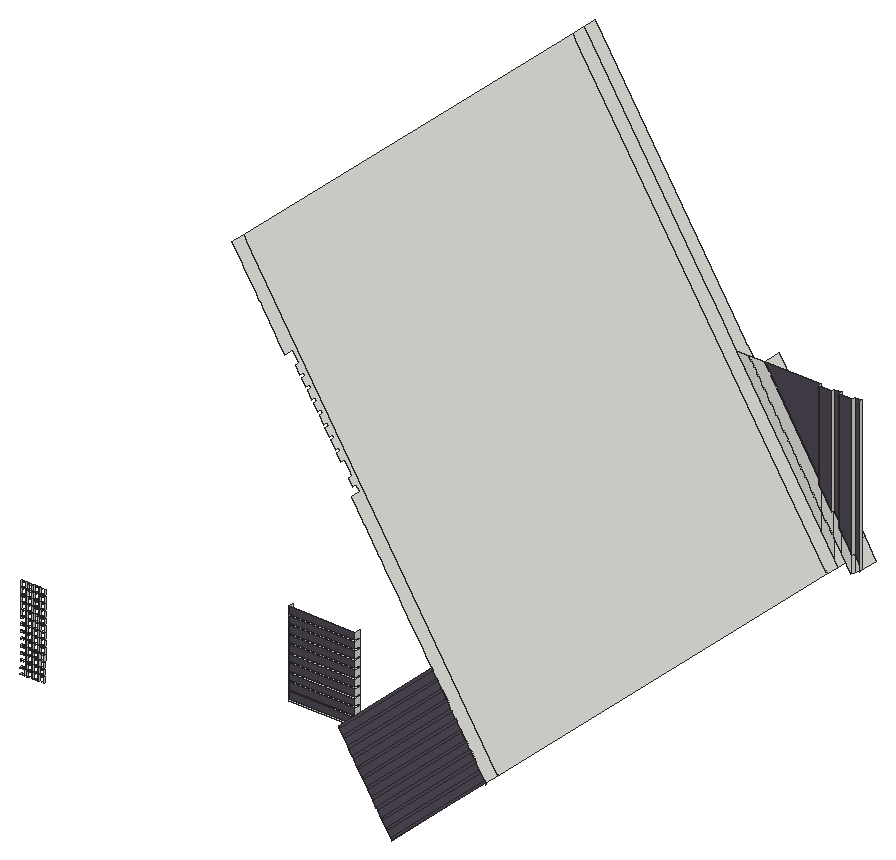
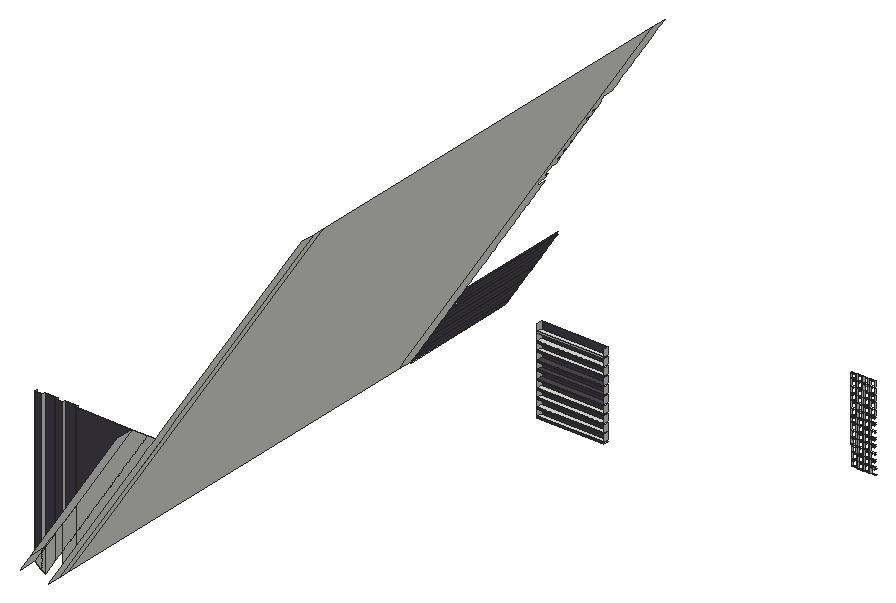
# SketchUp Ruby script. Lengths in inches.
U = 1.inch
M = Sketchup.active_model
def pt(a) = Geom::Point3d.new(a.map { |v| v * U })
def face(e, loops, mat)
  f = e.add_face(loops[0].map { |a| pt(a) })
  loops[1..].each { |l| e.add_face(l.map { |a| pt(a) }).erase! }
  f.material = f.back_material = mat if mat
  f
end
# faces: each face lists its corners as indices into pts; further lists are holes
def faces(e, pts, list, mat = nil) = list.each { |f| face(e, (f[0].is_a?(Array) ? f : [f]).map { |l| l.map { |i| pts[i] } }, mat) }
# xy, xz, yz: faces in a plane at the given z, y or x. An outline is a flat list of corners, or four numbers for a rectangle; further outlines are holes
def ring(l) = l.size == 4 ? [[l[0], l[1]], [l[2], l[1]], [l[2], l[3]], [l[0], l[3]]] : l.each_slice(2).to_a
def flat(e, list, mat, &to3) = list.each { |f| face(e, (f[0].is_a?(Array) ? f : [f]).map { |l| ring(l).map { |u, v| to3.(u, v) } }, mat) }
def xy(e, z, list, mat = nil) = flat(e, list, mat) { |x, y| [x, y, z] }
def xz(e, y, list, mat = nil) = flat(e, list, mat) { |x, z| [x, y, z] }
def yz(e, x, list, mat = nil) = flat(e, list, mat) { |y, z| [x, y, z] }
def lines(e, pts, list) = list.each { |a, b| e.add_line(pt(pts[a]), pt(pts[b])) }
# prism: a flat outline (further loops are holes) pulled along v
def prism(e, loops, v, mat = nil)
  f = face(e, loops, mat); d = Geom::Vector3d.new(v.map { |x| x * U })
  f.pushpull(f.normal.samedirection?(d) ? d.length : -d.length)
end
def box(e, o, s, mat = nil) = prism(e, [[o, [o[0] + s[0], o[1], o[2]], [o[0] + s[0], o[1] + s[1], o[2]], [o[0], o[1] + s[1], o[2]]]], [0, 0, s[2]], mat)
def at(x, y, z, deg = 0) = Geom::Transformation.translation(pt([x, y, z])) * Geom::Transformation.rotation(ORIGIN, Z_AXIS, deg.degrees)
def axes(o, x, y, z) = Geom::Transformation.new([*x, 0, *y, 0, *z, 0, *pt(o).to_a, 1])
def part(name) = M.definitions.add(name)
# library, detail: a bought-in or finely detailed component or shape, given as its bounding box
def library(name, o, s) = part(name).tap { |d| box(d.entities, o, s) }
def detail(e, o, s) = box(e.add_group.entities, o, s)
def put(e, d, t, mat = nil) = e.add_instance(d, t).tap { |i| i.material = mat if mat }
def group(e, t, mat = nil) = e.add_group.tap { |g| g.transformation = t; g.material = mat if mat }.entities
root = M.entities
M.materials.add("[Color M06]").color = [79, 71, 84]
xy(root,265.77,[[1006.85,2332.13,1009.17,2332.76],[1009.76,2332.13,1012.08,2332.76],[1012.68,2332.13,1014.99,2332.76],[1015.59,2332.13,1017.9,2332.76]])
xy(root,267.02,[[1096.79,2375.74,1127.76,2378.12]])
xy(root,267.83,[[1096.79,2375.74,1127.76,2378.12]])
xy(root,268.09,[[1006.85,2332.13,1009.17,2332.76],[1009.76,2332.13,1012.08,2332.76],[1012.68,2332.13,1014.99,2332.76],[1015.59,2332.13,1017.9,2332.76]])
xy(root,268.82,[[1006.88,2332.13,1009.19,2332.76],[1009.79,2332.13,1012.11,2332.76],[1012.71,2332.13,1015.02,2332.76],[1015.62,2332.13,1017.93,2332.76]])
xy(root,270.95,[[1096.79,2375.74,1127.76,2378.12]])
xy(root,271.13,[[1006.88,2332.13,1009.19,2332.76],[1009.79,2332.13,1012.11,2332.76],[1012.71,2332.13,1015.02,2332.76],[1015.62,2332.13,1017.93,2332.76]])
xy(root,271.76,[[1096.79,2375.74,1127.76,2378.12]])
xy(root,271.86,[[1006.91,2332.13,1009.22,2332.76],[1009.82,2332.13,1012.14,2332.76],[1012.73,2332.13,1015.05,2332.76],[1015.65,2332.13,1017.96,2332.76]])
xy(root,274.17,[[1006.91,2332.13,1009.22,2332.76],[1009.82,2332.13,1012.14,2332.76],[1012.73,2332.13,1015.05,2332.76],[1015.65,2332.13,1017.96,2332.76]])
xy(root,274.89,[[1096.79,2375.74,1127.76,2378.12]])
xy(root,274.91,[[1006.94,2332.13,1009.25,2332.76],[1009.85,2332.13,1012.16,2332.76],[1012.76,2332.13,1015.08,2332.76],[1015.68,2332.13,1017.99,2332.76]])
xy(root,275.7,[[1096.79,2375.74,1127.76,2378.12]])
xy(root,277.22,[[1006.94,2332.13,1009.25,2332.76],[1009.85,2332.13,1012.16,2332.76],[1012.76,2332.13,1015.08,2332.76],[1015.68,2332.13,1017.99,2332.76]])
xy(root,277.95,[[1006.97,2332.13,1009.28,2332.76],[1009.88,2332.13,1012.19,2332.76],[1012.79,2332.13,1015.11,2332.76],[1015.7,2332.13,1018.02,2332.76]])
xy(root,278.83,[[1096.79,2375.74,1127.76,2378.12]])
xy(root,279.64,[[1096.79,2375.74,1127.76,2378.12]])
xy(root,280.26,[[1006.97,2332.13,1009.28,2332.76],[1009.88,2332.13,1012.19,2332.76],[1012.79,2332.13,1015.11,2332.76],[1015.7,2332.13,1018.02,2332.76]])
xy(root,281,[[1007,2332.13,1009.31,2332.76],[1009.91,2332.13,1012.22,2332.76],[1012.82,2332.13,1015.13,2332.76],[1015.73,2332.13,1018.05,2332.76]])
xy(root,282.77,[[1096.79,2375.74,1127.76,2378.12]])
xy(root,283.31,[[1007,2332.13,1009.31,2332.76],[1009.91,2332.13,1012.22,2332.76],[1012.82,2332.13,1015.13,2332.76],[1015.73,2332.13,1018.05,2332.76]])
xy(root,283.58,[[1096.79,2375.74,1127.76,2378.12]],"[Color M06]")
xy(root,284.04,[[1007.03,2332.13,1009.34,2332.76],[1009.9375,2332.13,1012.25,2332.76],[1012.85,2332.13,1015.16,2332.76],[1015.76,2332.13,1018.08,2332.76]])
xy(root,286.35,[[1007.03,2332.13,1009.34,2332.76],[1009.9375,2332.13,1012.25,2332.76],[1012.85,2332.13,1015.16,2332.76],[1015.76,2332.13,1018.08,2332.76]])
xy(root,286.7,[[1096.79,2375.74,1127.76,2378.12]])
xy(root,287.09,[[1007.06,2332.13,1009.37,2332.76],[1009.97,2332.13,1012.28,2332.76],[1012.88,2332.13,1015.19,2332.76],[1015.79,2332.13,1018.1,2332.76]])
xy(root,287.51,[[1096.79,2375.74,1127.76,2378.12]],"[Color M06]")
xy(root,289.4,[[1007.06,2332.13,1009.37,2332.76],[1009.97,2332.13,1012.28,2332.76],[1012.88,2332.13,1015.19,2332.76],[1015.79,2332.13,1018.1,2332.76]])
xy(root,290.13,[[1007.08,2332.13,1009.4,2332.76],[1010,2332.13,1012.31,2332.76],[1012.91,2332.13,1015.22,2332.76],[1015.82,2332.13,1018.13,2332.76]])
xy(root,290.64,[[1096.79,2375.74,1127.76,2378.12]])
xy(root,291.45,[[1096.79,2375.74,1127.76,2378.12]],"[Color M06]")
xy(root,292.44,[[1007.08,2332.13,1009.4,2332.76],[1010,2332.13,1012.31,2332.76],[1012.91,2332.13,1015.22,2332.76],[1015.82,2332.13,1018.13,2332.76]])
xy(root,293.18,[[1007.11,2332.13,1009.43,2332.76],[1010.03,2332.13,1012.34,2332.76],[1012.9375,2332.13,1015.25,2332.76],[1015.85,2332.13,1018.16,2332.76]])
xy(root,294.58,[[1096.79,2375.74,1127.76,2378.12]])
xy(root,295.39,[[1096.79,2375.74,1127.76,2378.12]])
xy(root,295.49,[[1007.11,2332.13,1009.43,2332.76],[1010.03,2332.13,1012.34,2332.76],[1012.9375,2332.13,1015.25,2332.76],[1015.85,2332.13,1018.16,2332.76]])
xy(root,296.22,[[1007.14,2332.13,1009.46,2332.76],[1010.05,2332.13,1012.37,2332.76],[1012.97,2332.13,1015.28,2332.76],[1015.88,2332.13,1018.19,2332.76]])
xy(root,298.52,[[1096.79,2375.74,1127.76,2378.12]])
xy(root,298.53,[[1007.14,2332.13,1009.46,2332.76],[1010.05,2332.13,1012.37,2332.76],[1012.97,2332.13,1015.28,2332.76],[1015.88,2332.13,1018.19,2332.76]])
xy(root,299.27,[[1007.17,2332.13,1009.48,2332.76],[1010.08,2332.13,1012.4,2332.76],[1013,2332.13,1015.31,2332.76],[1015.91,2332.13,1018.22,2332.76]])
xy(root,299.33,[[1096.79,2375.74,1127.76,2378.12]])
xy(root,301.58,[[1007.17,2332.13,1009.48,2332.76],[1010.08,2332.13,1012.4,2332.76],[1013,2332.13,1015.31,2332.76],[1015.91,2332.13,1018.22,2332.76]])
xy(root,302.31,[[1007.2,2332.13,1009.51,2332.76],[1010.11,2332.13,1012.43,2332.76],[1013.02,2332.13,1015.34,2332.76],[1015.9375,2332.13,1018.25,2332.76]])
xy(root,302.45,[[1096.79,2375.74,1127.76,2378.12]])
xy(root,303.26,[[1096.79,2375.74,1127.76,2378.12]])
xy(root,304.62,[[1007.2,2332.13,1009.51,2332.76],[1010.11,2332.13,1012.43,2332.76],[1013.02,2332.13,1015.34,2332.76],[1015.9375,2332.13,1018.25,2332.76]])
xz(root,2373.56,[[1190.19,265.95,1189.93,266.36,1190.19,266.53],[1189.4,267.19,1189.66,267.36,1187.96,270,1187.7,269.84],[1187.17,270.67,1187.43,270.83,1185.74,273.48,1185.48,273.31],[1184.94,274.14,1185.21,274.31,1183.51,276.95,1183.25,276.78],[1182.72,277.61,1182.98,277.78,1181.29,280.42,1181.02,280.25],
  [1180.49,281.08,1180.75,281.25,1179.06,283.89,1178.8,283.73],[1178.26,284.56,1178.53,284.72,1176.83,287.37,1176.57,287.2],[1176.04,288.03,1176.3,288.2,1174.61,290.84,1174.34,290.67],[1173.8125,291.5,1172.12,294.14,1172.38,294.3125,1174.07,291.67],[1171.59,294.97,1171.85,295.14,1170.15,297.79,1169.89,297.62],
  [1169.36,298.45,1169.62,298.61,1167.93,301.26,1167.66,301.09],[1167.03,301.85,1167.4,302.09,1165.7,304.73,1165.33,304.49]])
xz(root,2375.74,[[1096.79,267.83,1127.76,270.95],[1096.79,271.76,1127.76,274.89],[1096.79,275.7,1127.76,278.83],[1096.79,279.64,1127.76,282.77],[1096.79,283.58,1127.76,286.7],
  [1096.79,287.51,1127.76,290.64],[1096.79,291.45,1127.76,294.58],[1096.79,295.39,1127.76,298.52],[1096.79,299.33,1127.76,302.45],[1096.79,303.26,1127.76,306.39]],"[Color M06]")
xz(root,2378.12,[[1096.79,302.45,1127.76,303.26]])
xz(root,2378.12,[[1096.79,267.02,1127.76,267.83],[1096.79,270.95,1127.76,271.76],[1096.79,274.89,1127.76,275.7],[1096.79,278.83,1127.76,279.64],[1096.79,282.77,1127.76,283.58],
  [1096.79,286.7,1127.76,287.51],[1096.79,290.64,1127.76,291.45],[1096.79,294.58,1127.76,295.39],[1096.79,298.52,1127.76,299.33]],"[Color M06]")
xz(root,2576.81,[[1198,274.85,1198,340.125,1191.92,340.125,1191.92,284.33,1196.26,277.56],[1188.5,289.67,1188.5,340.125,1182.42,340.125,1182.42,299.15]],"[Color M06]")
xz(root,2578.12,[[1196.26,265.98,1196.26,277.56,1191.92,284.33,1191.92,272.75],[1196.26,265.98,1198,267.09,1198,274.85,1196.26,277.56],[1198,267.09,1198,274.85,1201.42,269.51,1201.42,269.29],[1188.5,269.17,1188.5,278.09,1182.42,287.57,1182.42,278.65],[1201.42,269.29,1201.52,269.35,1201.42,269.51],
  [1191.92,272.75,1191.92,284.33,1188.5,289.67,1188.5,278.09],[1188.5,278.09,1188.5,289.67,1182.42,299.15,1182.42,287.57],[1182.42,278.65,1182.42,287.57,1148.73,340.125,1143.01,340.125],[1182.42,287.57,1182.42,299.15,1156.15,340.125,1148.73,340.125]])
xz(root,2578.12,[[1201.42,269.51,1201.42,340.125,1198,340.125,1198,274.85],[1191.92,284.33,1191.92,340.125,1188.5,340.125,1188.5,289.67],[1182.42,299.15,1182.42,340.125,1156.15,340.125]],"[Color M06]")
yz(root,1007.08,[[2332.13,290.13,2332.76,292.44]])
yz(root,1007.11,[[2332.13,293.18,2332.76,295.49]])
yz(root,1007.14,[[2332.13,296.22,2332.76,298.53]])
yz(root,1007.17,[[2332.13,299.27,2332.76,301.58]])
yz(root,1007.2,[[2332.13,302.31,2332.76,304.62]])
yz(root,1009.17,[[2332.13,265.77,2332.76,268.09]])
yz(root,1009.19,[[2332.13,268.82,2332.76,271.13]])
yz(root,1009.22,[[2332.13,271.86,2332.76,274.17]])
yz(root,1009.25,[[2332.13,274.91,2332.76,277.22]])
yz(root,1009.28,[[2332.13,277.95,2332.76,280.26]])
yz(root,1009.31,[[2332.13,281,2332.76,283.31]])
yz(root,1009.34,[[2332.13,284.04,2332.76,286.35]])
yz(root,1009.37,[[2332.13,287.09,2332.76,289.4]])
yz(root,1009.4,[[2332.13,290.13,2332.76,292.44]])
yz(root,1009.43,[[2332.13,293.18,2332.76,295.49]])
yz(root,1009.46,[[2332.13,296.22,2332.76,298.53]])
yz(root,1009.48,[[2332.13,299.27,2332.76,301.58]])
yz(root,1009.51,[[2332.13,302.31,2332.76,304.62]])
yz(root,1009.76,[[2332.13,265.77,2332.76,268.09]])
yz(root,1009.79,[[2332.13,268.82,2332.76,271.13]])
yz(root,1009.82,[[2332.13,271.86,2332.76,274.17]])
yz(root,1009.85,[[2332.13,274.91,2332.76,277.22]])
yz(root,1009.88,[[2332.13,277.95,2332.76,280.26]])
yz(root,1009.91,[[2332.13,281,2332.76,283.31]])
yz(root,1009.9375,[[2332.13,284.04,2332.76,286.35]])
yz(root,1009.97,[[2332.13,287.09,2332.76,289.4]])
yz(root,1010,[[2332.13,290.13,2332.76,292.44]])
yz(root,1010.03,[[2332.13,293.18,2332.76,295.49]])
yz(root,1010.05,[[2332.13,296.22,2332.76,298.53]])
yz(root,1010.08,[[2332.13,299.27,2332.76,301.58]])
yz(root,1010.11,[[2332.13,302.31,2332.76,304.62]])
yz(root,1012.08,[[2332.13,265.77,2332.76,268.09]])
yz(root,1012.11,[[2332.13,268.82,2332.76,271.13]])
yz(root,1012.14,[[2332.13,271.86,2332.76,274.17]])
yz(root,1012.16,[[2332.13,274.91,2332.76,277.22]])
yz(root,1012.19,[[2332.13,277.95,2332.76,280.26]])
yz(root,1012.22,[[2332.13,281,2332.76,283.31]])
yz(root,1012.25,[[2332.13,284.04,2332.76,286.35]])
yz(root,1012.28,[[2332.13,287.09,2332.76,289.4]])
yz(root,1012.31,[[2332.13,290.13,2332.76,292.44]])
yz(root,1012.34,[[2332.13,293.18,2332.76,295.49]])
yz(root,1012.37,[[2332.13,296.22,2332.76,298.53]])
yz(root,1012.4,[[2332.13,299.27,2332.76,301.58]])
yz(root,1012.43,[[2332.13,302.31,2332.76,304.62]])
yz(root,1012.68,[[2332.13,265.77,2332.76,268.09]])
yz(root,1012.71,[[2332.13,268.82,2332.76,271.13]])
yz(root,1012.73,[[2332.13,271.86,2332.76,274.17]])
yz(root,1012.76,[[2332.13,274.91,2332.76,277.22]])
yz(root,1012.79,[[2332.13,277.95,2332.76,280.26]])
yz(root,1012.82,[[2332.13,281,2332.76,283.31]])
yz(root,1012.85,[[2332.13,284.04,2332.76,286.35]])
yz(root,1012.88,[[2332.13,287.09,2332.76,289.4]])
yz(root,1012.91,[[2332.13,290.13,2332.76,292.44]])
yz(root,1012.9375,[[2332.13,293.18,2332.76,295.49]])
yz(root,1012.97,[[2332.13,296.22,2332.76,298.53]])
yz(root,1013,[[2332.13,299.27,2332.76,301.58]])
yz(root,1013.02,[[2332.13,302.31,2332.76,304.62]])
yz(root,1014.99,[[2332.13,265.77,2332.76,268.09]])
yz(root,1015.02,[[2332.13,268.82,2332.76,271.13]])
yz(root,1015.05,[[2332.13,271.86,2332.76,274.17]])
yz(root,1015.08,[[2332.13,274.91,2332.76,277.22]])
yz(root,1015.11,[[2332.13,277.95,2332.76,280.26]])
yz(root,1015.13,[[2332.13,281,2332.76,283.31]])
yz(root,1015.16,[[2332.13,284.04,2332.76,286.35]])
yz(root,1015.19,[[2332.13,287.09,2332.76,289.4]])
yz(root,1015.22,[[2332.13,290.13,2332.76,292.44]])
yz(root,1015.25,[[2332.13,293.18,2332.76,295.49]])
yz(root,1015.28,[[2332.13,296.22,2332.76,298.53]])
yz(root,1015.31,[[2332.13,299.27,2332.76,301.58]])
yz(root,1015.34,[[2332.13,302.31,2332.76,304.62]])
yz(root,1015.59,[[2332.13,265.77,2332.76,268.09]])
yz(root,1015.62,[[2332.13,268.82,2332.76,271.13]])
yz(root,1015.65,[[2332.13,271.86,2332.76,274.17]])
yz(root,1015.68,[[2332.13,274.91,2332.76,277.22]])
yz(root,1015.7,[[2332.13,277.95,2332.76,280.26]])
yz(root,1015.73,[[2332.13,281,2332.76,283.31]])
yz(root,1015.76,[[2332.13,284.04,2332.76,286.35]])
yz(root,1015.79,[[2332.13,287.09,2332.76,289.4]])
yz(root,1015.82,[[2332.13,290.13,2332.76,292.44]])
yz(root,1015.85,[[2332.13,293.18,2332.76,295.49]])
yz(root,1015.88,[[2332.13,296.22,2332.76,298.53]])
yz(root,1015.91,[[2332.13,299.27,2332.76,301.58]])
yz(root,1015.9375,[[2332.13,302.31,2332.76,304.62]])
yz(root,1017.9,[[2332.13,265.77,2332.76,268.09]])
yz(root,1017.93,[[2332.13,268.82,2332.76,271.13]])
yz(root,1017.96,[[2332.13,271.86,2332.76,274.17]])
yz(root,1017.99,[[2332.13,274.91,2332.76,277.22]])
yz(root,1018.02,[[2332.13,277.95,2332.76,280.26]])
yz(root,1018.05,[[2332.13,281,2332.76,283.31]])
yz(root,1018.08,[[2332.13,284.04,2332.76,286.35]])
yz(root,1018.1,[[2332.13,287.09,2332.76,289.4]])
yz(root,1018.13,[[2332.13,290.13,2332.76,292.44]])
yz(root,1018.16,[[2332.13,293.18,2332.76,295.49]])
yz(root,1018.19,[[2332.13,296.22,2332.76,298.53]])
yz(root,1018.22,[[2332.13,299.27,2332.76,301.58]])
yz(root,1018.25,[[2332.13,302.31,2332.76,304.62]])
yz(root,1096.79,[[2375.74,267.83,2378.12,270.95],[2375.74,271.76,2378.12,274.89],[2375.74,275.7,2378.12,278.83],[2375.74,279.64,2378.12,282.77],[2375.74,283.58,2378.12,286.7],
  [2375.74,287.51,2378.12,290.64],[2375.74,291.45,2378.12,294.58],[2375.74,295.39,2378.12,298.52],[2375.74,299.33,2378.12,302.45],[2375.74,303.26,2378.12,306.39]])
yz(root,1127.76,[[2375.74,267.83,2378.12,270.95],[2375.74,271.76,2378.12,274.89],[2375.74,275.7,2378.12,278.83],[2375.74,279.64,2378.12,282.77],[2375.74,283.58,2378.12,286.7],
  [2375.74,287.51,2378.12,290.64],[2375.74,291.45,2378.12,294.58],[2375.74,295.39,2378.12,298.52],[2375.74,299.33,2378.12,302.45],[2375.74,303.26,2378.12,306.39]])
yz(root,1182.42,[[2576.81,299.15,2578.12,340.125]])
yz(root,1188.5,[[2576.81,289.67,2578.12,340.125]])
yz(root,1191.92,[[2576.81,284.33,2578.12,340.125]])
yz(root,1198,[[2576.81,274.85,2578.12,340.125]])
yz(root,1201.42,[[2576.81,269.51,2578.12,340.125]])
p = [[1190.19,2319.18,266.53],[1190.19,2373.56,266.53],[1189.93,2373.56,266.36],[1189.93,2319.18,266.36],[1189.66,2319.18,267.36],[1189.66,2373.56,267.36],
  [1190.19,2380.48,266.53],[1072.29,2380.48,450.4375],[1072.29,2373.56,450.4375],[1072.67,2373.56,449.84],[1073.86,2373.56,447.99],[1074.41,2373.56,447.125],
  [1074.86,2373.56,446.42],[1076.05,2373.56,444.57],[1076.6,2373.56,443.7],[1077.05,2373.56,443],[1078.24,2373.56,441.15],[1078.8,2373.56,440.28],
  [1079.25,2373.56,439.58],[1080.43,2373.56,437.73],[1080.99,2373.56,436.86],[1081.4375,2373.56,436.16],[1082.625,2373.56,434.31],[1083.18,2373.56,433.44],
  [1083.63,2373.56,432.74],[1084.82,2373.56,430.89],[1085.375,2373.56,430.02],[1085.82,2373.56,429.32],[1087.01,2373.56,427.47],[1087.57,2373.56,426.6],
  [1088.02,2373.56,425.9],[1089.2,2373.56,424.05],[1089.76,2373.56,423.18],[1090.21,2373.56,422.48],[1091.4,2373.56,420.63],[1091.95,2373.56,419.76],
  [1092.4,2373.56,419.0625],[1093.59,2373.56,417.21],[1094.14,2373.56,416.34],[1094.59,2373.56,415.64],[1095.78,2373.56,413.79],[1096.34,2373.56,412.92],
  [1096.79,2373.56,412.22],[1096.79,2378.12,412.22],[1096.85,2378.12,412.12],[1098.86,2378.12,409],[1099.74,2378.12,407.62],[1099.74,2376.24,407.62],
  [1101.74,2376.24,404.5],[1101.74,2378.12,404.5],[1102.46,2378.12,403.37],[1102.46,2376.24,403.37],[1104.47,2376.24,400.25],[1104.47,2378.12,400.25],
  [1105.1875,2378.12,399.12],[1105.1875,2376.24,399.12],[1107.19,2376.24,396],[1107.19,2378.12,396],[1107.91,2378.12,394.87],[1107.91,2376.24,394.87],
  [1109.92,2376.24,391.75],[1109.92,2378.12,391.75],[1110.64,2378.12,390.62],[1110.64,2376.24,390.62],[1112.64,2376.24,387.5],[1112.64,2378.12,387.5],
  [1113.36,2378.12,386.37],[1113.36,2376.24,386.37],[1115.36,2376.24,383.25],[1115.36,2378.12,383.25],[1116.08,2378.12,382.12],[1116.08,2376.24,382.12],
  [1118.09,2376.24,379],[1118.09,2378.12,379],[1118.81,2378.12,377.87],[1118.81,2376.24,377.87],[1120.8125,2376.24,374.75],[1120.8125,2378.12,374.75],
  [1121.53,2378.12,373.62],[1123.54,2378.12,370.5],[1124.26,2378.12,369.37],[1124.26,2376.24,369.37],[1126.26,2376.24,366.25],[1126.26,2378.12,366.25],
  [1126.98,2378.12,365.12],[1127.76,2378.12,363.92],[1127.76,2376.24,363.92],[1127.76,2373.56,363.92],[1128.94,2373.56,362.07],[1129.57,2373.56,361.08],
  [1129.63,2373.56,360.99],[1131.27,2373.56,358.4375],[1131.9,2373.56,357.45],[1133.6,2373.56,354.81],[1134.23,2373.56,353.82],[1135.92,2373.56,351.18],
  [1136.56,2373.56,350.19],[1138.25,2373.56,347.55],[1138.88,2373.56,346.56],[1140.58,2373.56,343.92],[1141.21,2373.56,342.93],[1142.91,2373.56,340.29],
  [1143.01,2373.56,340.125],[1143.4375,2373.56,339.46],[1145.13,2373.56,336.8125],[1145.66,2373.56,335.98],[1147.36,2373.56,333.34],[1147.89,2373.56,332.51],
  [1149.59,2373.56,329.87],[1150.12,2373.56,329.04],[1151.8125,2373.56,326.4],[1152.34,2373.56,325.57],[1154.04,2373.56,322.92],[1154.57,2373.56,322.09],
  [1156.26,2373.56,319.45],[1156.8,2373.56,318.62],[1158.49,2373.56,315.98],[1159.02,2373.56,315.15],[1160.72,2373.56,312.51],[1161.25,2373.56,311.68],
  [1162.94,2373.56,309.03],[1163.47,2373.56,308.2],[1165.17,2373.56,305.56],[1165.7,2373.56,304.73],[1167.4,2373.56,302.09],[1167.93,2373.56,301.26],
  [1169.62,2373.56,298.61],[1170.15,2373.56,297.79],[1171.85,2373.56,295.14],[1172.38,2373.56,294.3125],[1174.07,2373.56,291.67],[1174.61,2373.56,290.84],
  [1176.3,2373.56,288.2],[1176.83,2373.56,287.37],[1178.53,2373.56,284.72],[1179.06,2373.56,283.89],[1180.75,2373.56,281.25],[1181.29,2373.56,280.42],
  [1182.98,2373.56,277.78],[1183.51,2373.56,276.95],[1185.21,2373.56,274.31],[1185.74,2373.56,273.48],[1187.43,2373.56,270.83],[1187.96,2373.56,270],
  [1190.19,2571.59,266.53],[1072.29,2571.59,450.4375],[1143.01,2578.12,340.125],[1182.42,2578.12,278.65],[1188.5,2578.12,269.17],[1190.19,2578.12,266.53],
  [1072.29,2578.12,450.4375],[1127.1,2578.12,364.9375],[1130.09,2578.12,360.28],[1136.56,2578.12,350.1875],[1072.29,2583.74,450.4375],[1190.19,2584.2,266.53],
  [1150.78,2584.2,328],[1149.7,2584.2,329.69],[1143.8125,2584.2,338.875],[1143.01,2584.2,340.125],[1142.28,2584.2,341.27],[1136.56,2584.2,350.1875],
  [1072.29,2584.2,450.4375],[1187.7,2373.56,269.84],[1189.4,2373.56,267.19],[1189.4,2319.18,267.19],[1187.7,2319.18,269.84],[1201.52,2578.12,269.35],
  [1201.42,2578.12,269.51],[1201.42,2576.81,269.51],[1201.52,2576.81,269.35],[1198,2578.12,274.85],[1196.26,2578.12,277.56],[1196.26,2586.43,277.56],
  [1201.52,2586.43,269.35],[1187.96,2319.18,270],[1187.43,2319.18,270.83],[1185.48,2373.56,273.31],[1187.17,2373.56,270.67],[1187.17,2319.18,270.67],
  [1185.48,2319.18,273.31],[1185.74,2319.18,273.48],[1185.21,2319.18,274.31],[1183.25,2373.56,276.78],[1184.94,2373.56,274.14],[1184.94,2319.18,274.14],
  [1183.25,2319.18,276.78],[1196.26,2576.81,277.56],[1198,2576.81,274.85],[1183.51,2319.18,276.95],[1182.98,2319.18,277.78],[1181.02,2373.56,280.25],
  [1182.72,2373.56,277.61],[1182.72,2319.18,277.61],[1181.02,2319.18,280.25],[1191.92,2578.12,284.33],[1191.92,2576.81,284.33],[1182.42,2578.12,299.15],
  [1156.15,2578.12,340.125],[1156.15,2584.2,340.125],[1156.15,2586.43,340.125],[1188.5,2578.12,289.67],[1181.29,2319.18,280.42],[1180.75,2319.18,281.25],
  [1178.8,2373.56,283.73],[1180.49,2373.56,281.08],[1180.49,2319.18,281.08],[1178.8,2319.18,283.73],[1179.06,2319.18,283.89],[1178.53,2319.18,284.72],
  [1176.57,2373.56,287.2],[1178.26,2373.56,284.56],[1178.26,2319.18,284.56],[1176.57,2319.18,287.2],[1176.83,2319.18,287.37],[1176.3,2319.18,288.2],
  [1174.34,2373.56,290.67],[1176.04,2373.56,288.03],[1176.04,2319.18,288.03],[1174.34,2319.18,290.67],[1182.42,2576.81,299.15],[1188.5,2576.81,289.67],
  [1174.61,2319.18,290.84],[1174.07,2319.18,291.67],[1172.12,2373.56,294.14],[1173.8125,2373.56,291.5],[1173.8125,2319.18,291.5],[1172.12,2319.18,294.14],
  [1172.38,2319.18,294.3125],[1171.85,2319.18,295.14],[1169.89,2373.56,297.62],[1171.59,2373.56,294.97],[1171.59,2319.18,294.97],[1169.89,2319.18,297.62],
  [1170.15,2319.18,297.79],[1169.62,2319.18,298.61],[1167.66,2373.56,301.09],[1169.36,2373.56,298.45],[1169.36,2319.18,298.45],[1167.66,2319.18,301.09],
  [1167.93,2319.18,301.26],[1167.4,2319.18,302.09],[1165.33,2373.56,304.49],[1167.03,2373.56,301.85],[1167.03,2319.18,301.85],[1165.33,2319.18,304.49],
  [1165.7,2319.18,304.73],[1165.17,2319.18,305.56]]
faces(root,p,[[0,1,2,3],[6,7,8,9,10,11,12,13,14,15,16,17,18,19,20,21,22,23,24,25,26,27,28,29,30,31,32,33,34,35,36,37,38,39,40,41,42,43,44,45,46,47,48,49,50,51,52,53,54,55,56,57,58,59,60,61,62,63,64,65,66,67,68,69,70,71,72,73,74,75,76,77,78,79,80,81,82,83,84,85,86,87,88,89,90,91,92,93,94,95,96,97,98,99,100,101,102,103,104,105,106,107,108,109,110,111,112,113,114,115,116,117,118,119,120,121,122,123,124,125,126,127,128,129,130,131,132,133,134,135,136,137,138,139,140,141,142,143,5,1],[144,6,7,145],[146,147,148,149,144,145,150,151,152,153],[154,150,151,152,153,146,147,148,149,155,156,157,158,159,160,161,162],[5,4,165,164],[167,168,169,170],[171,172,173,174,167,168],
  [175,143,163,166],[142,176,179,178],[181,141,177,180],[140,182,185,184],[171,172,187,188],[189,139,183,186],[138,190,193,192],[172,195,196,187],
  [197,198,199,200,173,172,195,201],[202,137,191,194],[136,203,206,205],[208,135,204,207],[134,209,212,211],[214,133,210,213],[132,215,218,217],[201,197,220,221],
  [222,131,216,219],[130,223,226,225],[228,129,224,227],[128,229,232,231],[234,127,230,233],[126,235,238,237],[240,125,236,239],[124,241,244,243],
  [246,123,242,245]])
faces(root,p,[[0,4,5,1],[163,164,165,166],[175,176,142,143],[177,178,179,180],[181,182,140,141],[183,184,185,186],[189,190,138,139],[191,192,193,194],
  [202,203,136,137],[204,205,206,207],[208,209,134,135],[210,211,212,213],[214,215,132,133],[216,217,218,219],[222,223,130,131],[224,225,226,227],
  [228,229,128,129],[230,231,232,233],[234,235,126,127],[236,237,238,239],[240,241,124,125],[242,243,244,245],[246,247,122,123]],"[Color M06]")
